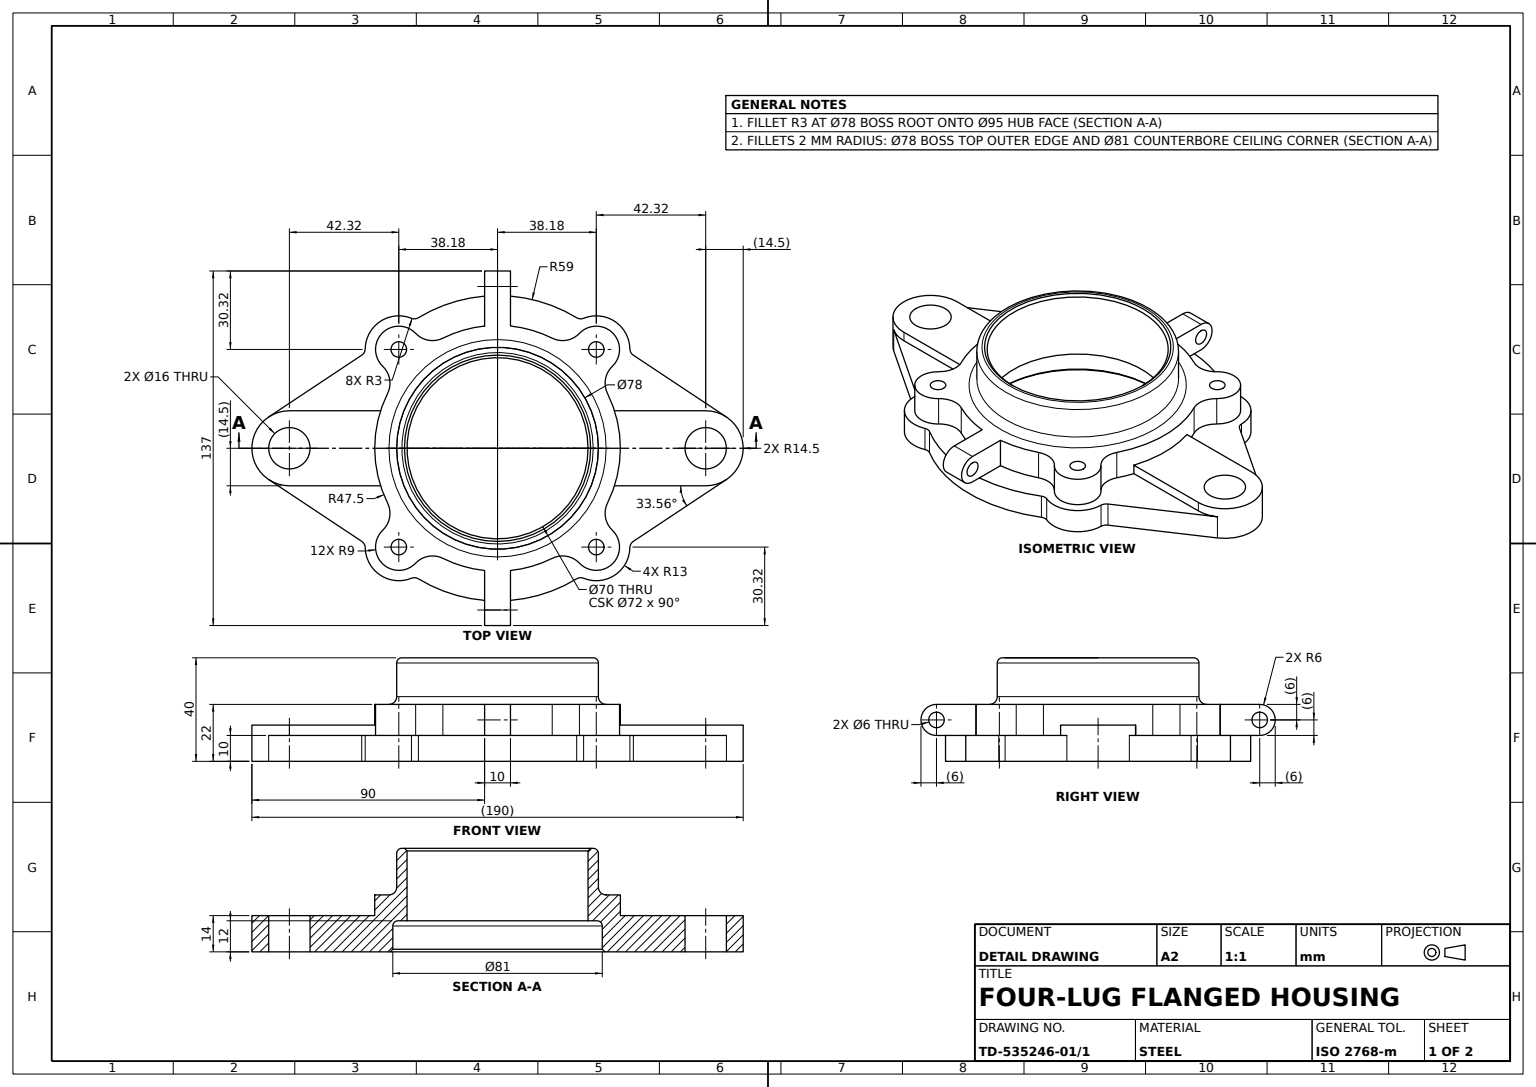
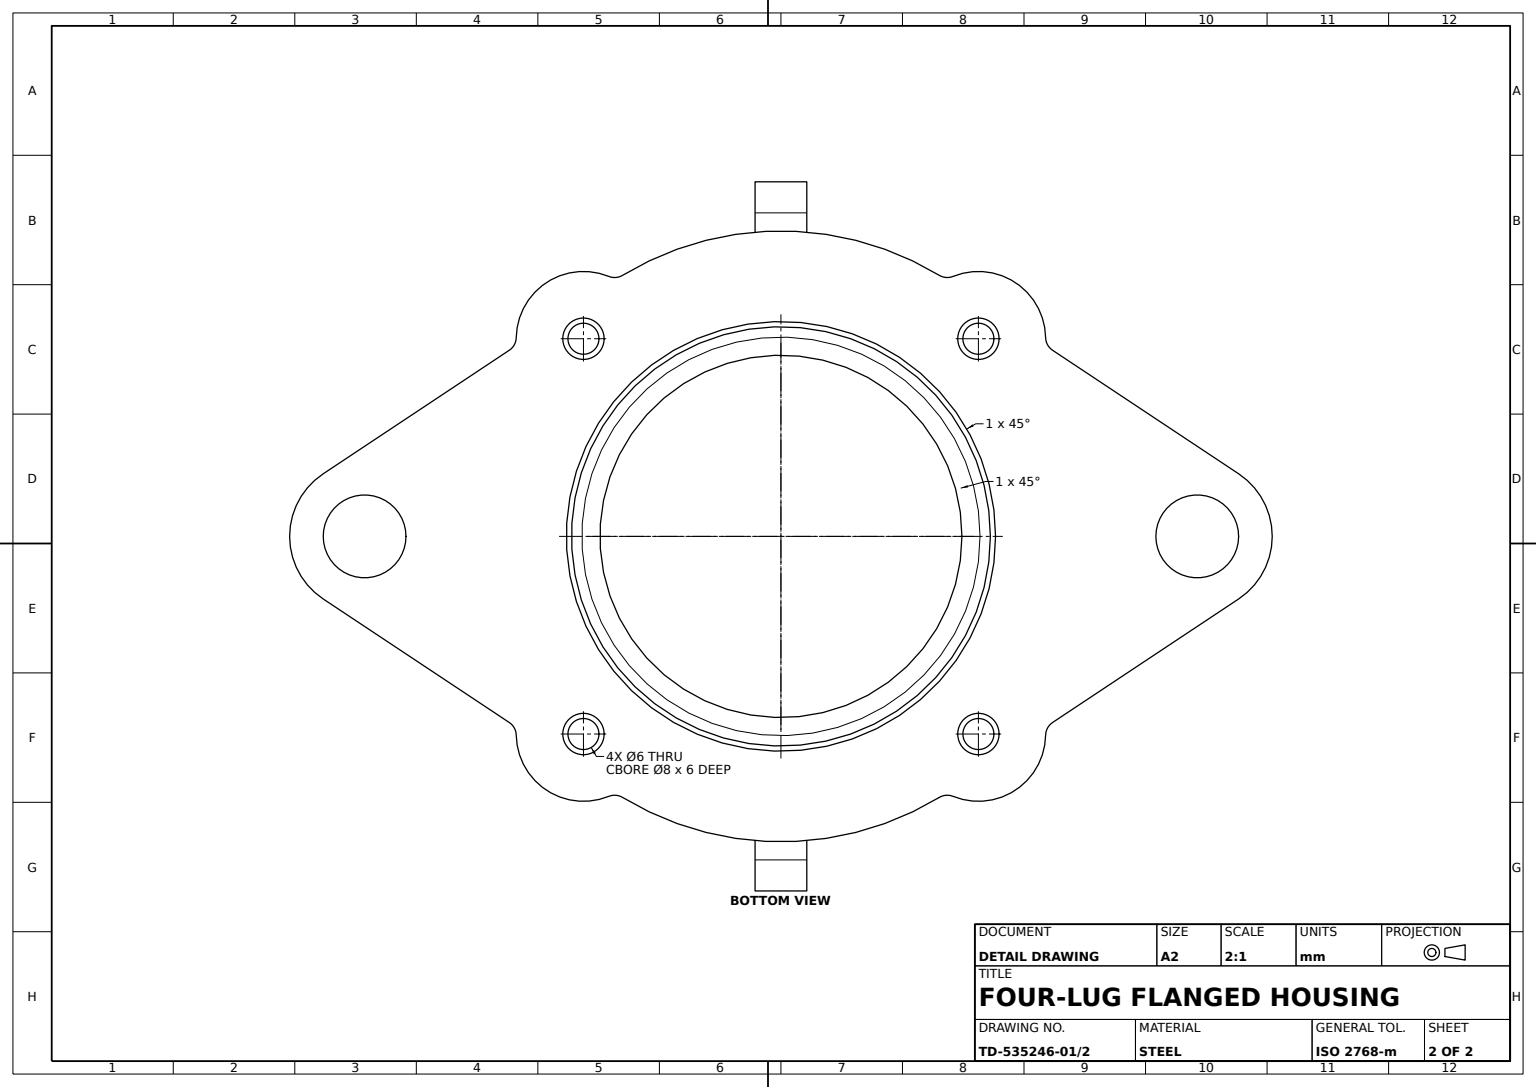
solid
v1 (42.183766,-38.183766,6)
e1 v1 v1 CIRCLE(AX(P(38.183766,-38.183766,6),D(0,0,1),D(1,0,0)),4) rev
v2 (42.183766,-38.183766,0)
e2 v2 v2 CIRCLE(AX(P(38.183766,-38.183766,0),D(0,0,1),D(1,0,0)),4)
face CYL(AX(P(38.183766,-38.183766,0),D(0,0,1),D(1,0,0)),4) rev [-e1] [-e2]
v3 (-35.183766,-38.183766,22)
e3 v3 v3 CIRCLE(AX(P(-38.183766,-38.183766,22),D(0,0,1),D(1,0,0)),3)
v4 (-35.183766,-38.183766,6)
e4 v4 v4 CIRCLE(AX(P(-38.183766,-38.183766,6),D(0,0,1),D(1,0,0)),3) rev
face CYL(AX(P(-38.183766,-38.183766,139.020471),D(0,0,1),D(1,0,0)),3) rev [e3] [e4]
v5 (31.665409,44.389491,22)
v6 (21.141326,42.5358,22)
e5 v5 v6 CIRCLE(AX(P(25.147051,50.595215,22),D(0,0,1),D(1,0,0)),9) rev
v7 (31.665409,44.389491,10)
e6 v7 v5 LINE
v8 (21.141326,42.5358,10)
e7 v8 v7 CIRCLE(AX(P(25.147051,50.595215,10),D(0,0,1),D(1,0,0)),9)
e8 v6 v8 LINE
face CYL(AX(P(25.147051,50.595215,22),D(0,0,-1),D(-1,0,0)),9) rev [-e5 -e6 -e7 -e8]
v9 (-51.181838,-38.407634,0)
v10 (-52.523009,-35.959344,0)
e9 v9 v10 CIRCLE(AX(P(-54.181394,-38.459296,0),D(0,0,1),D(1,0,0)),3)
v11 (-51.181838,-38.407634,10)
e10 v11 v9 LINE
v12 (-52.523009,-35.959344,10)
e11 v12 v11 CIRCLE(AX(P(-54.181394,-38.459296,10),D(0,0,1),D(1,0,0)),3) rev
e12 v10 v12 LINE
face CYL(AX(P(-54.181394,-38.459296,10),D(0,0,-1),D(-1,0,0)),3) rev [-e9 -e10 -e11 -e12]
v13 (5,-62.5,10)
v14 (-5,-62.5,10)
e13 v13 v14 LINE
v15 (5,-62.5,22)
e14 v13 v15 CIRCLE(AX(P(5,-62.5,16),D(-1,0,0),D(0,1,0)),6)
v16 (-5,-62.5,22)
e15 v15 v16 LINE
e16 v14 v16 CIRCLE(AX(P(-5,-62.5,16),D(-1,0,0),D(0,1,0)),6)
face CYL(AX(P(5,-62.5,16),D(-1,0,0),D(0,0,1)),6) [-e13 e14 e15 -e16]
v17 (42,0,22)
e17 v17 v17 CIRCLE(AX(P(0,0,22),D(0,0,1),D(1,0,0)),42) rev
v18 (39,0,25)
e18 v18 v18 CIRCLE(AX(P(0,0,25),D(0,0,1),D(1,0,0)),39)
face TORUS(AX(P(0,0,25),D(0,0,1),D(1,0,0)),42,3) rev [-e17] [-e18]
v19 (5,62.5,19)
e19 v19 v19 CIRCLE(AX(P(5,62.5,16),D(-1,0,0),D(0,0,1)),3)
v20 (5,47.236109,10)
v21 (5,47.236109,22)
e20 v20 v21 LINE
v22 (5,58.787754,10)
e21 v20 v22 LINE
v23 (5,62.5,10)
e22 v22 v23 LINE
v24 (5,62.5,22)
e23 v23 v24 CIRCLE(AX(P(5,62.5,16),D(1,0,0),D(0,-1,0)),6)
e24 v24 v21 LINE
face PLANE(AX(P(5,62.5,16),D(1,0,0),D(0,0,-1))) [e19] [-e20 e21 e22 e23 e24]
v25 (-80.5,-14.5,14)
v26 (-80.5,-14.5,10)
e25 v25 v26 LINE
v27 (-45.232732,-14.5,10)
e26 v27 v26 LINE
v28 (-45.232732,-14.5,14)
e27 v28 v27 LINE
e28 v25 v28 LINE
face PLANE(AX(P(-80.5,-14.5,14),D(0,1,0),D(0,0,1))) rev [e25 -e26 -e27 -e28]
v29 (-44.389491,-31.665409,22)
v30 (-31.665409,-44.389491,22)
e29 v29 v30 CIRCLE(AX(P(-38.183766,-38.183766,22),D(0,0,1),D(0,1,0)),9)
v31 (-44.389491,-31.665409,10)
e30 v29 v31 LINE
v32 (-31.665409,-44.389491,10)
e31 v32 v31 CIRCLE(AX(P(-38.183766,-38.183766,10),D(0,0,1),D(1,0,0)),9) rev
e32 v32 v30 LINE
face CYL(AX(P(-38.183766,-38.183766,22),D(0,0,-1),D(-1,0,0)),9) [-e29 e30 -e31 e32]
v33 (-88.515528,-12.0831,0)
e33 v33 v10 LINE
v34 (-88.515528,-12.0831,10)
e34 v34 v12 LINE
e35 v34 v33 LINE
face PLANE(AX(P(-88.515528,-12.0831,10),D(0.552795031,0.833317259,0),D(-0.833317259,0.552795031,0))) rev [e33 e12 -e34 e35]
v35 (35,0,12)
e36 v35 v35 CIRCLE(AX(P(0,0,12),D(0,0,1),D(1,0,0)),35) rev
v36 (38.5,0,12)
e37 v36 v36 CIRCLE(AX(P(0,0,12),D(0,0,1),D(1,0,0)),38.5) rev
face PLANE(AX(P(0,0,12),D(0,0,1),D(1,0,0))) rev [-e36] [e37]
v37 (88.5,0,0)
e38 v37 v37 CIRCLE(AX(P(80.5,0,0),D(0,0,1),D(1,0,0)),8)
v38 (72.5,0,14)
e39 v38 v38 CIRCLE(AX(P(80.5,0,14),D(0,0,-1),D(-1,0,0)),8)
face CYL(AX(P(80.5,0,14),D(0,0,-1),D(-1,0,0)),8) rev [-e38] [-e39]
v39 (51.181838,38.407634,10)
v40 (51.181838,38.407634,0)
e40 v39 v40 LINE
v41 (52.523009,35.959344,10)
e41 v41 v39 CIRCLE(AX(P(54.181394,38.459296,10),D(0,0,1),D(1,0,0)),3) rev
v42 (52.523009,35.959344,0)
e42 v42 v41 LINE
e43 v40 v42 CIRCLE(AX(P(54.181394,38.459296,0),D(0,0,1),D(1,0,0)),3)
face CYL(AX(P(54.181394,38.459296,10),D(0,0,-1),D(-1,0,0)),3) rev [-e40 -e41 -e42 -e43]
v43 (-33.289778,-50.22739,10)
e44 v11 v43 CIRCLE(AX(P(-38.183766,-38.183766,10),D(0,0,1),D(0,1,0)),13)
v44 (-33.289778,-50.22739,0)
e45 v9 v44 CIRCLE(AX(P(-38.183766,-38.183766,0),D(0,0,1),D(0,1,0)),13)
e46 v44 v43 LINE
face CYL(AX(P(-38.183766,-38.183766,10),D(0,0,-1),D(-1,0,0)),13) [-e44 e10 e45 e46]
v45 (-51.181838,38.407634,10)
v46 (-52.523009,35.959344,10)
e47 v45 v46 CIRCLE(AX(P(-54.181394,38.459296,10),D(0,0,1),D(1,0,0)),3) rev
v47 (-51.181838,38.407634,0)
e48 v47 v45 LINE
v48 (-52.523009,35.959344,0)
e49 v48 v47 CIRCLE(AX(P(-54.181394,38.459296,0),D(0,0,1),D(1,0,0)),3)
e50 v46 v48 LINE
face CYL(AX(P(-54.181394,38.459296,10),D(0,0,-1),D(-1,0,0)),3) rev [-e47 -e48 -e49 -e50]
v49 (39,0,38)
e51 v49 v49 CIRCLE(AX(P(0,0,38),D(0,0,1),D(1,0,0)),39) rev
face CYL(AX(P(0,0,40),D(0,0,-1),D(-1,0,0)),39) [e51] [e18]
v50 (-42.5358,-21.141326,22)
e52 v50 v29 CIRCLE(AX(P(-50.595215,-25.147051,22),D(0,0,1),D(1,0,0)),9) rev
v51 (-42.5358,-21.141326,10)
e53 v51 v50 LINE
e54 v31 v51 CIRCLE(AX(P(-50.595215,-25.147051,10),D(0,0,1),D(1,0,0)),9)
face CYL(AX(P(-50.595215,-25.147051,22),D(0,0,1),D(1,0,0)),9) rev [-e52 -e53 -e54 -e30]
v52 (33.289778,-50.22739,10)
v53 (33.289778,-50.22739,0)
e55 v52 v53 LINE
v54 (30.604247,-50.441848,10)
e56 v54 v52 CIRCLE(AX(P(32.160396,-53.006688,10),D(0,0,1),D(1,0,0)),3) rev
v55 (30.604247,-50.441848,0)
e57 v55 v54 LINE
e58 v53 v55 CIRCLE(AX(P(32.160396,-53.006688,0),D(0,0,1),D(1,0,0)),3)
face CYL(AX(P(32.160396,-53.006688,10),D(0,0,1),D(1,0,0)),3) rev [-e55 -e56 -e57 -e58]
v56 (40.5,0,1)
e59 v56 v56 CIRCLE(AX(P(0,0,1),D(0,0,1),D(1,0,0)),40.5) rev
v57 (40.5,0,10)
e60 v57 v57 CIRCLE(AX(P(0,0,10),D(0,0,1),D(1,0,0)),40.5)
face CYL(AX(P(0,0,0),D(0,0,1),D(1,0,0)),40.5) rev [e59] [e60]
v58 (42.183766,38.183766,0)
e61 v58 v58 CIRCLE(AX(P(38.183766,38.183766,0),D(0,0,1),D(1,0,0)),4)
v59 (41.5,0,0)
e62 v59 v59 CIRCLE(AX(P(0,0,0),D(0,0,1),D(1,0,0)),41.5)
v60 (-34.183766,-38.183766,0)
e63 v60 v60 CIRCLE(AX(P(-38.183766,-38.183766,0),D(0,0,1),D(1,0,0)),4)
v61 (-72.5,0,0)
e64 v61 v61 CIRCLE(AX(P(-80.5,0,0),D(0,0,1),D(1,0,0)),8)
v62 (-34.183766,38.183766,0)
e65 v62 v62 CIRCLE(AX(P(-38.183766,38.183766,0),D(0,0,1),D(1,0,0)),4)
v63 (88.515528,12.0831,0)
e66 v63 v42 LINE
v64 (88.515528,-12.0831,0)
e67 v64 v63 CIRCLE(AX(P(80.5,0,0),D(0,0,1),D(1,0,0)),14.5)
v65 (52.523009,-35.959344,0)
e68 v65 v64 LINE
v66 (51.181838,-38.407634,0)
e69 v65 v66 CIRCLE(AX(P(54.181394,-38.459296,0),D(0,0,1),D(1,0,0)),3)
e70 v53 v66 CIRCLE(AX(P(38.183766,-38.183766,0),D(0,0,1),D(-1,0,0)),13)
v67 (-30.604247,-50.441848,0)
e71 v67 v55 CIRCLE(AX(P(0,0,0),D(0,0,1),D(1,0,0)),59)
e72 v67 v44 CIRCLE(AX(P(-32.160396,-53.006688,0),D(0,0,1),D(1,0,0)),3)
v68 (-88.515528,12.0831,0)
e73 v68 v33 CIRCLE(AX(P(-80.5,0,0),D(0,0,1),D(1,0,0)),14.5)
e74 v48 v68 LINE
v69 (-33.289778,50.22739,0)
e75 v69 v47 CIRCLE(AX(P(-38.183766,38.183766,0),D(0,0,1),D(1,0,0)),13)
v70 (-30.604247,50.441848,0)
e76 v69 v70 CIRCLE(AX(P(-32.160396,53.006688,0),D(0,0,1),D(1,0,0)),3)
v71 (30.604247,50.441848,0)
e77 v71 v70 CIRCLE(AX(P(0,0,0),D(0,0,1),D(1,0,0)),59)
v72 (33.289778,50.22739,0)
e78 v71 v72 CIRCLE(AX(P(32.160396,53.006688,0),D(0,0,1),D(1,0,0)),3)
e79 v40 v72 CIRCLE(AX(P(38.183766,38.183766,0),D(0,0,1),D(0,-1,0)),13)
face PLANE(AX(P(0,0,0),D(0,0,1),D(1,0,0))) rev [e61] [e2] [e62] [e63] [e64] [e65] [e43 -e66 -e67 -e68 e69 -e70 e58 -e71 e72 -e45 e9 -e33 -e73 -e74 e49 -e75 e76 -e77 e78 -e79] [e38]
v73 (42.5358,-21.141326,22)
v74 (42.5358,-21.141326,10)
e80 v73 v74 LINE
v75 (44.389491,-31.665409,22)
e81 v75 v73 CIRCLE(AX(P(50.595215,-25.147051,22),D(0,0,1),D(1,0,0)),9) rev
v76 (44.389491,-31.665409,10)
e82 v76 v75 LINE
e83 v74 v76 CIRCLE(AX(P(50.595215,-25.147051,10),D(0,0,1),D(1,0,0)),9)
face CYL(AX(P(50.595215,-25.147051,22),D(0,0,-1),D(-1,0,0)),9) rev [-e80 -e81 -e82 -e83]
v77 (-88.515528,12.0831,10)
e84 v77 v68 LINE
e85 v46 v77 LINE
face PLANE(AX(P(-32.614907,49.165718,10),D(0.552795031,-0.833317259,0),D(0.833317259,0.552795031,0))) rev [e50 e74 -e84 -e85]
v78 (-5,-58.787754,10)
v79 (5,-58.787754,10)
e86 v78 v79 CIRCLE(AX(P(0,0,10),D(0,0,1),D(1,0,0)),59)
e87 v79 v13 LINE
e88 v78 v14 LINE
face PLANE(AX(P(5,-43.900041,10),D(0,0,-1),D(-1,0,0))) [e86 e87 e13 -e88]
v80 (41.183766,38.183766,22)
e89 v80 v80 CIRCLE(AX(P(38.183766,38.183766,22),D(0,0,1),D(1,0,0)),3)
v81 (41.183766,38.183766,6)
e90 v81 v81 CIRCLE(AX(P(38.183766,38.183766,6),D(0,0,1),D(1,0,0)),3) rev
face CYL(AX(P(38.183766,38.183766,139.020471),D(0,0,1),D(1,0,0)),3) rev [e89] [e90]
v82 (51.181838,-38.407634,10)
e91 v66 v82 LINE
e92 v52 v82 CIRCLE(AX(P(38.183766,-38.183766,10),D(0,0,1),D(-1,0,0)),13)
face CYL(AX(P(38.183766,-38.183766,10),D(0,0,-1),D(-1,0,0)),13) [e70 e91 -e92 e55]
v83 (-33.289778,50.22739,10)
e93 v83 v45 CIRCLE(AX(P(-38.183766,38.183766,10),D(0,0,1),D(1,0,0)),13)
e94 v83 v69 LINE
face CYL(AX(P(-38.183766,38.183766,10),D(0,0,-1),D(-1,0,0)),13) [-e93 e94 e75 e48]
v84 (35,0,39)
e95 v84 v84 CIRCLE(AX(P(0,0,39),D(0,0,1),D(1,0,0)),35)
face CYL(AX(P(0,0,150.697638),D(0,0,1),D(1,0,0)),35) rev [e95] [e36]
v85 (-80.5,14.5,10)
e96 v77 v85 CIRCLE(AX(P(-80.5,0,10),D(0,0,1),D(1,0,0)),14.5) rev
v86 (-45.232732,14.5,10)
e97 v85 v86 LINE
v87 (-42.5358,21.141326,10)
e98 v86 v87 CIRCLE(AX(P(0,0,10),D(0,0,1),D(1,0,0)),47.5) rev
v88 (-44.389491,31.665409,10)
e99 v87 v88 CIRCLE(AX(P(-50.595215,25.147051,10),D(0,0,1),D(1,0,0)),9)
v89 (-31.665409,44.389491,10)
e100 v88 v89 CIRCLE(AX(P(-38.183766,38.183766,10),D(0,0,1),D(1,0,0)),9) rev
v90 (-21.141326,42.5358,10)
e101 v89 v90 CIRCLE(AX(P(-25.147051,50.595215,10),D(0,0,1),D(1,0,0)),9)
v91 (-5,47.236109,10)
e102 v90 v91 CIRCLE(AX(P(0,0,10),D(0,0,1),D(1,0,0)),47.5) rev
v92 (-5,58.787754,10)
e103 v91 v92 LINE
v93 (-30.604247,50.441848,10)
e104 v92 v93 CIRCLE(AX(P(0,0,10),D(0,0,1),D(1,0,0)),59)
e105 v93 v83 CIRCLE(AX(P(-32.160396,53.006688,10),D(0,0,1),D(1,0,0)),3) rev
face PLANE(AX(P(0,0,10),D(0,0,1),D(1,0,0))) [e96 e97 e98 e99 e100 e101 e102 e103 e104 e105 e93 e47 e85]
v94 (5,-62.5,19)
e106 v94 v94 CIRCLE(AX(P(5,-62.5,16),D(-1,0,0),D(0,0,1)),3)
v95 (-5,-62.5,19)
e107 v95 v95 CIRCLE(AX(P(-5,-62.5,16),D(-1,0,0),D(0,0,1)),3)
face CYL(AX(P(5,-62.5,16),D(-1,0,0),D(0,0,1)),3) rev [-e106] [e107]
v96 (-44.389491,31.665409,22)
e108 v88 v96 LINE
v97 (-31.665409,44.389491,22)
e109 v97 v96 CIRCLE(AX(P(-38.183766,38.183766,22),D(0,0,1),D(1,0,0)),9)
e110 v97 v89 LINE
face CYL(AX(P(-38.183766,38.183766,22),D(0,0,-1),D(-1,0,0)),9) [e108 -e109 e110 -e100]
v98 (45.232732,14.5,14)
v99 (80.5,14.5,14)
e111 v98 v99 LINE
v100 (80.5,14.5,10)
e112 v99 v100 LINE
v101 (45.232732,14.5,10)
e113 v100 v101 LINE
e114 v98 v101 LINE
face PLANE(AX(P(45.232732,14.5,14),D(0,1,0),D(0,0,1))) [e111 e112 e113 -e114]
v102 (21.141326,-42.5358,10)
v103 (5,-47.236109,10)
e115 v102 v103 CIRCLE(AX(P(0,0,10),D(0,0,1),D(1,0,0)),47.5) rev
e116 v103 v79 LINE
e117 v79 v54 CIRCLE(AX(P(0,0,10),D(0,0,1),D(1,0,0)),59)
v104 (52.523009,-35.959344,10)
e118 v82 v104 CIRCLE(AX(P(54.181394,-38.459296,10),D(0,0,1),D(1,0,0)),3) rev
v105 (88.515528,-12.0831,10)
e119 v104 v105 LINE
v106 (80.5,-14.5,10)
e120 v105 v106 CIRCLE(AX(P(80.5,0,10),D(0,0,1),D(1,0,0)),14.5) rev
v107 (45.232732,-14.5,10)
e121 v107 v106 LINE
e122 v107 v74 CIRCLE(AX(P(0,0,10),D(0,0,1),D(1,0,0)),47.5) rev
v108 (31.665409,-44.389491,10)
e123 v76 v108 CIRCLE(AX(P(38.183766,-38.183766,10),D(0,0,1),D(1,0,0)),9) rev
e124 v108 v102 CIRCLE(AX(P(25.147051,-50.595215,10),D(0,0,1),D(1,0,0)),9)
face PLANE(AX(P(0,0,10),D(0,0,1),D(1,0,0))) [e115 e116 e117 e56 e92 e118 e119 e120 -e121 e122 e83 e123 e124]
e125 v70 v93 LINE
face CYL(AX(P(-32.160396,53.006688,10),D(0,0,1),D(1,0,0)),3) rev [-e76 -e94 -e105 -e125]
v109 (-45.232732,14.5,14)
v110 (-80.5,14.5,14)
e126 v109 v110 LINE
e127 v109 v86 LINE
e128 v110 v85 LINE
face PLANE(AX(P(-45.232732,14.5,14),D(0,-1,0),D(0,0,-1))) rev [-e126 e127 -e97 -e128]
v111 (-21.141326,-42.5358,22)
e129 v30 v111 CIRCLE(AX(P(-25.147051,-50.595215,22),D(0,0,1),D(1,0,0)),9) rev
v112 (-21.141326,-42.5358,10)
e130 v112 v32 CIRCLE(AX(P(-25.147051,-50.595215,10),D(0,0,1),D(1,0,0)),9)
e131 v111 v112 LINE
face CYL(AX(P(-25.147051,-50.595215,22),D(0,0,-1),D(-1,0,0)),9) rev [-e129 -e32 -e130 -e131]
v113 (42.183766,38.183766,6)
e132 v113 v113 CIRCLE(AX(P(38.183766,38.183766,6),D(0,0,1),D(1,0,0)),4) rev
face CYL(AX(P(38.183766,38.183766,0),D(0,0,1),D(1,0,0)),4) rev [-e132] [-e61]
v114 (44.389491,31.665409,22)
v115 (44.389491,31.665409,10)
e133 v114 v115 LINE
e134 v7 v115 CIRCLE(AX(P(38.183766,38.183766,10),D(0,0,1),D(1,0,0)),9) rev
e135 v114 v5 CIRCLE(AX(P(38.183766,38.183766,22),D(0,0,1),D(0,-1,0)),9)
face CYL(AX(P(38.183766,38.183766,22),D(0,0,-1),D(-1,0,0)),9) [e133 -e134 e6 -e135]
v116 (5,-47.236109,22)
v117 (21.141326,-42.5358,22)
e136 v116 v117 CIRCLE(AX(P(0,0,22),D(0,0,1),D(1,0,0)),47.5)
e137 v103 v116 LINE
e138 v102 v117 LINE
face CYL(AX(P(0,0,22),D(0,0,-1),D(-1,0,0)),47.5) [-e136 -e137 -e115 e138]
v118 (-42.5358,21.141326,22)
e139 v118 v87 LINE
e140 v96 v118 CIRCLE(AX(P(-50.595215,25.147051,22),D(0,0,1),D(1,0,0)),9) rev
face CYL(AX(P(-50.595215,25.147051,22),D(0,0,-1),D(-1,0,0)),9) rev [-e99 -e139 -e140 -e108]
v119 (88.515528,12.0831,10)
e141 v119 v41 LINE
e142 v119 v63 LINE
face PLANE(AX(P(88.515528,12.0831,10),D(-0.552795031,-0.833317259,0),D(0.833317259,-0.552795031,0))) rev [-e141 e142 e66 e42]
e143 v26 v34 CIRCLE(AX(P(-80.5,0,10),D(0,0,1),D(1,0,0)),14.5) rev
e144 v110 v25 CIRCLE(AX(P(-80.5,0,14),D(0,0,1),D(1,0,0)),14.5)
face CYL(AX(P(-80.5,0,10),D(0,0,-1),D(-1,0,0)),14.5) [e84 e73 -e35 -e143 -e25 -e144 e128 -e96]
v120 (-30.604247,-50.441848,10)
e145 v120 v78 CIRCLE(AX(P(0,0,10),D(0,0,1),D(1,0,0)),59)
e146 v120 v67 LINE
face CYL(AX(P(0,0,10),D(0,0,-1),D(-1,0,0)),59) [e57 -e117 -e86 -e145 e146 e71]
v121 (-34.183766,-38.183766,6)
e147 v121 v121 CIRCLE(AX(P(-38.183766,-38.183766,6),D(0,0,1),D(1,0,0)),4) rev
face PLANE(AX(P(-38.183766,-38.183766,6),D(0,0,1),D(1,0,0))) rev [-e4] [e147]
v122 (41.183766,-38.183766,22)
e148 v122 v122 CIRCLE(AX(P(38.183766,-38.183766,22),D(0,0,1),D(1,0,0)),3)
v123 (41.183766,-38.183766,6)
e149 v123 v123 CIRCLE(AX(P(38.183766,-38.183766,6),D(0,0,1),D(1,0,0)),3) rev
face CYL(AX(P(38.183766,-38.183766,139.020471),D(0,0,1),D(1,0,0)),3) rev [e148] [e149]
v124 (-34.183766,38.183766,6)
e150 v124 v124 CIRCLE(AX(P(-38.183766,38.183766,6),D(0,0,1),D(1,0,0)),4) rev
v125 (-35.183766,38.183766,6)
e151 v125 v125 CIRCLE(AX(P(-38.183766,38.183766,6),D(0,0,1),D(1,0,0)),3) rev
face PLANE(AX(P(-38.183766,38.183766,6),D(0,0,1),D(1,0,0))) rev [e150] [-e151]
v126 (42.5358,21.141326,22)
e152 v126 v114 CIRCLE(AX(P(50.595215,25.147051,22),D(0,0,1),D(1,0,0)),9) rev
v127 (42.5358,21.141326,10)
e153 v127 v126 LINE
e154 v115 v127 CIRCLE(AX(P(50.595215,25.147051,10),D(0,0,1),D(1,0,0)),9)
face CYL(AX(P(50.595215,25.147051,22),D(0,0,1),D(1,0,0)),9) rev [-e152 -e153 -e154 -e133]
v128 (-5,-47.236109,10)
e155 v128 v78 LINE
v129 (-5,-47.236109,22)
e156 v16 v129 LINE
e157 v128 v129 LINE
face PLANE(AX(P(-5,-62.5,16),D(-1,0,0),D(0,0,1))) [e155 e88 e16 e156 -e157] [-e107]
v130 (36,0,40)
e158 v130 v130 CIRCLE(AX(P(0,0,40),D(0,0,1),D(1,0,0)),36) rev
face CONE(AX(P(0,0,39),D(0,0,1),D(1,0,0)),35,0.785398163) rev [-e158] [-e95]
v131 (-21.141326,42.5358,22)
e159 v131 v97 CIRCLE(AX(P(-25.147051,50.595215,22),D(0,0,1),D(1,0,0)),9) rev
e160 v90 v131 LINE
face CYL(AX(P(-25.147051,50.595215,22),D(0,0,1),D(1,0,0)),9) rev [-e101 -e110 -e159 -e160]
e161 v22 v92 CIRCLE(AX(P(0,0,10),D(0,0,1),D(1,0,0)),59)
v132 (-5,62.5,10)
e162 v92 v132 LINE
e163 v23 v132 LINE
face PLANE(AX(P(5,43.900041,10),D(0,0,1),D(1,0,0))) rev [e161 e162 -e163 -e22]
face PLANE(AX(P(38.183766,38.183766,6),D(0,0,1),D(1,0,0))) rev [-e90] [e132]
face CONE(AX(P(0,0,0),D(0,0,-1),D(-1,0,0)),41.5,0.785398163) rev [-e59] [-e62]
v133 (31.665409,-44.389491,22)
e164 v133 v75 CIRCLE(AX(P(38.183766,-38.183766,22),D(0,0,1),D(-1,0,0)),9)
e165 v133 v108 LINE
face CYL(AX(P(38.183766,-38.183766,22),D(0,0,-1),D(-1,0,0)),9) [-e164 e165 -e123 e82]
e166 v43 v120 CIRCLE(AX(P(-32.160396,-53.006688,10),D(0,0,1),D(1,0,0)),3) rev
face CYL(AX(P(-32.160396,-53.006688,10),D(0,0,-1),D(-1,0,0)),3) rev [-e72 -e146 -e166 -e46]
e167 v128 v112 CIRCLE(AX(P(0,0,10),D(0,0,1),D(1,0,0)),47.5) rev
e168 v51 v27 CIRCLE(AX(P(0,0,10),D(0,0,1),D(1,0,0)),47.5) rev
face PLANE(AX(P(0,0,10),D(0,0,1),D(1,0,0))) [e11 e44 e166 e145 -e155 e167 e130 e31 e54 e168 e26 e143 e34]
v134 (33.289778,50.22739,10)
e169 v72 v134 LINE
v135 (30.604247,50.441848,10)
e170 v135 v71 LINE
e171 v134 v135 CIRCLE(AX(P(32.160396,53.006688,10),D(0,0,1),D(1,0,0)),3) rev
face CYL(AX(P(32.160396,53.006688,10),D(0,0,-1),D(-1,0,0)),3) rev [-e169 -e78 -e170 -e171]
v136 (37,0,40)
e172 v136 v136 CIRCLE(AX(P(0,0,40),D(0,0,1),D(1,0,0)),37)
face PLANE(AX(P(0,0,40),D(0,0,1),D(1,0,0))) [e172] [e158]
e173 v20 v8 CIRCLE(AX(P(0,0,10),D(0,0,1),D(1,0,0)),47.5) rev
e174 v6 v21 CIRCLE(AX(P(0,0,22),D(0,0,1),D(1,0,0)),47.5)
face CYL(AX(P(0,0,22),D(0,0,-1),D(-1,0,0)),47.5) [-e173 e20 -e174 e8]
e175 v28 v109 CIRCLE(AX(P(0,0,14),D(0,0,-1),D(1,0,0)),47.5)
v137 (-88.5,0,14)
e176 v137 v137 CIRCLE(AX(P(-80.5,0,14),D(0,0,-1),D(-1,0,0)),8)
face PLANE(AX(P(-80.5,0,14),D(0,0,1),D(1,0,0))) [e175 e126 e144 e28] [e176]
e177 v135 v22 CIRCLE(AX(P(0,0,10),D(0,0,1),D(1,0,0)),59)
face CYL(AX(P(0,0,10),D(0,0,-1),D(-1,0,0)),59) [e170 e77 e125 -e104 -e161 -e177]
e178 v100 v119 CIRCLE(AX(P(80.5,0,10),D(0,0,1),D(1,0,0)),14.5) rev
v138 (80.5,-14.5,14)
e179 v99 v138 CIRCLE(AX(P(80.5,0,14),D(0,0,-1),D(-1,0,0)),14.5)
e180 v138 v106 LINE
e181 v105 v64 LINE
face CYL(AX(P(80.5,0,10),D(0,0,-1),D(-1,0,0)),14.5) [e67 -e142 -e178 -e112 e179 e180 -e120 e181]
face CYL(AX(P(-80.5,0,14),D(0,0,-1),D(-1,0,0)),8) rev [-e176] [-e64]
face PLANE(AX(P(38.183766,-38.183766,6),D(0,0,1),D(1,0,0))) rev [-e149] [e1]
e182 v39 v134 CIRCLE(AX(P(38.183766,38.183766,10),D(0,0,1),D(0,-1,0)),13)
face CYL(AX(P(38.183766,38.183766,10),D(0,0,-1),D(-1,0,0)),13) [e40 e79 e169 -e182]
e183 v118 v50 CIRCLE(AX(P(0,0,22),D(0,0,1),D(1,0,0)),47.5)
face CYL(AX(P(0,0,22),D(0,0,-1),D(-1,0,0)),47.5) [e53 -e183 e139 -e98 -e127 -e175 e27 -e168]
v139 (-5,47.236109,22)
e184 v139 v131 CIRCLE(AX(P(0,0,22),D(0,0,1),D(1,0,0)),47.5)
e185 v91 v139 LINE
face CYL(AX(P(0,0,22),D(0,0,-1),D(-1,0,0)),47.5) [e160 -e184 -e185 -e102]
e186 v127 v101 CIRCLE(AX(P(0,0,10),D(0,0,1),D(1,0,0)),47.5) rev
face PLANE(AX(P(0,0,10),D(0,0,1),D(1,0,0))) [-e21 e173 e7 e134 e154 e186 -e113 e178 e141 e41 e182 e171 e177]
e187 v104 v65 LINE
face CYL(AX(P(54.181394,-38.459296,10),D(0,0,-1),D(-1,0,0)),3) rev [-e187 -e118 -e91 -e69]
v140 (-5,62.5,13)
e188 v140 v140 CIRCLE(AX(P(-5,62.5,16),D(1,0,0),D(0,0,-1)),3)
v141 (-5,62.5,22)
e189 v141 v139 LINE
e190 v132 v141 CIRCLE(AX(P(-5,62.5,16),D(1,0,0),D(0,-1,0)),6)
face PLANE(AX(P(-5,62.5,16),D(1,0,0),D(0,0,-1))) rev [e188] [-e189 -e190 -e162 -e103 e185]
face CYL(AX(P(-38.183766,-38.183766,0),D(0,0,1),D(1,0,0)),4) rev [-e147] [-e63]
v142 (45.232732,-14.5,14)
e191 v138 v142 LINE
e192 v142 v107 LINE
face PLANE(AX(P(80.5,-14.5,14),D(0,-1,0),D(0,0,-1))) [-e180 e191 e192 e121]
v143 (-35.183766,38.183766,22)
e193 v143 v143 CIRCLE(AX(P(-38.183766,38.183766,22),D(0,0,1),D(1,0,0)),3)
face CYL(AX(P(-38.183766,38.183766,139.020471),D(0,0,1),D(1,0,0)),3) rev [e193] [e151]
face TORUS(AX(P(0,0,38),D(0,0,1),D(1,0,0)),37,2) [-e51] [-e172]
e194 v142 v98 CIRCLE(AX(P(0,0,14),D(0,0,1),D(-1,0,0)),47.5)
face PLANE(AX(P(80.5,0,14),D(0,0,-1),D(-1,0,0))) rev [e39] [-e191 -e179 -e111 -e194]
e195 v111 v129 CIRCLE(AX(P(0,0,22),D(0,0,1),D(1,0,0)),47.5)
face CYL(AX(P(0,0,22),D(0,0,-1),D(-1,0,0)),47.5) [-e195 e131 -e167 e157]
face CYL(AX(P(-38.183766,38.183766,0),D(0,0,1),D(1,0,0)),4) rev [-e150] [-e65]
e196 v117 v133 CIRCLE(AX(P(25.147051,-50.595215,22),D(0,0,1),D(1,0,0)),9) rev
face CYL(AX(P(25.147051,-50.595215,22),D(0,0,1),D(1,0,0)),9) rev [-e165 -e196 -e138 -e124]
e197 v73 v126 CIRCLE(AX(P(0,0,22),D(0,0,1),D(1,0,0)),47.5)
face CYL(AX(P(0,0,22),D(0,0,-1),D(-1,0,0)),47.5) [-e186 e153 -e197 e80 -e122 -e192 e194 e114]
e198 v24 v141 LINE
face CYL(AX(P(5,62.5,16),D(-1,0,0),D(0,0,1)),6) [e190 -e198 -e23 e163]
e199 v15 v116 LINE
face PLANE(AX(P(0,0,22),D(0,0,1),D(1,0,0))) [e17] [-e148] [-e3] [-e89] [-e156 -e15 e199 e136 e196 e164 e81 e197 e152 e135 e5 e174 -e24 e198 e189 e184 e159 e109 e140 e183 e52 e29 e129 e195] [-e193]
face TORUS(AX(P(0,0,10),D(0,0,1),D(1,0,0)),38.5,2) rev [-e37] [-e60]
face CYL(AX(P(5,62.5,16),D(-1,0,0),D(0,0,1)),3) rev [-e188] [-e19]
face PLANE(AX(P(5,-62.5,16),D(-1,0,0),D(0,0,1))) rev [e106] [-e199 -e14 -e87 -e116 e137]
face PLANE(AX(P(32.614907,-49.165718,10),D(-0.552795031,0.833317259,0),D(-0.833317259,-0.552795031,0))) rev [e68 -e181 -e119 e187]
